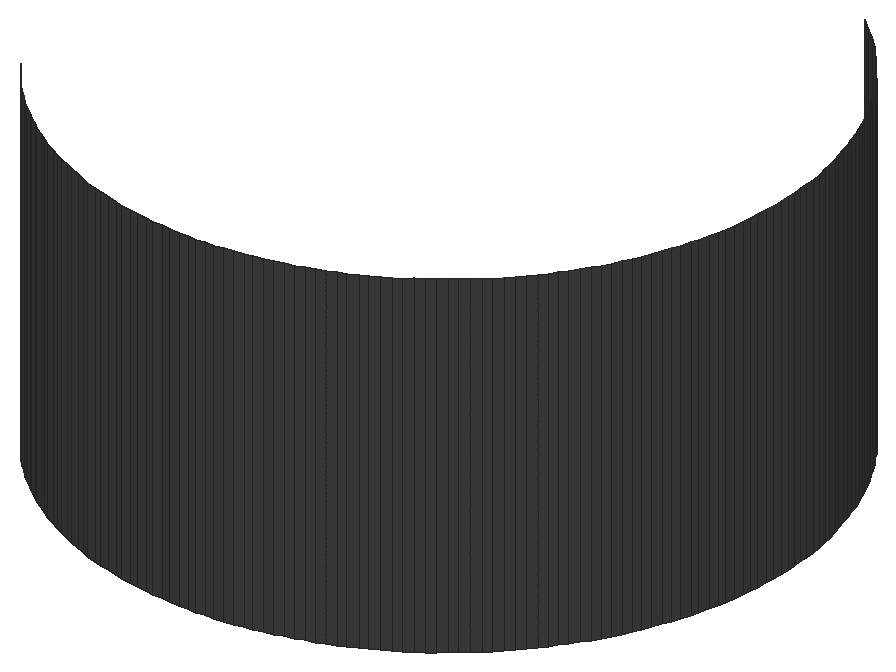
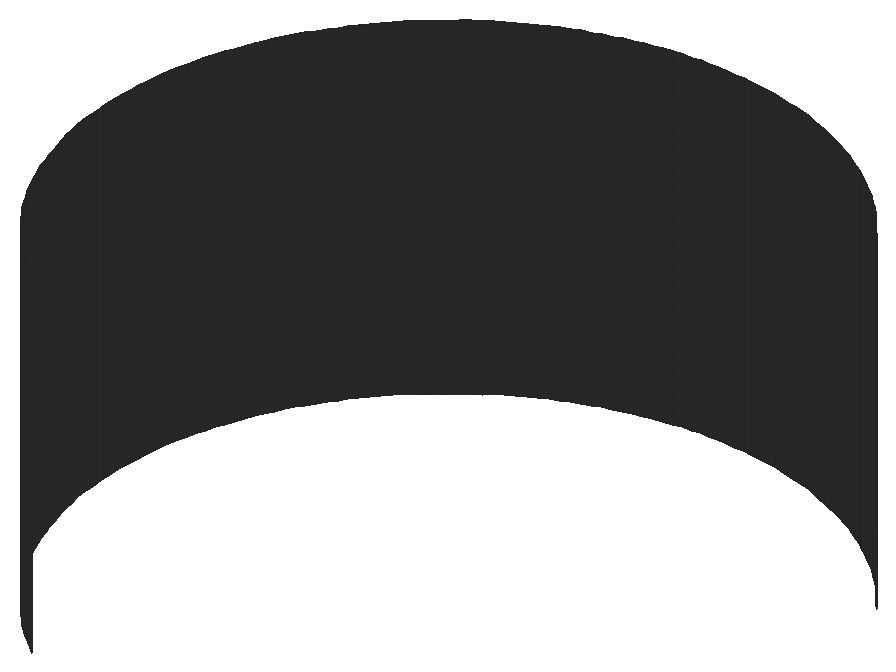
# SketchUp Ruby script. Lengths in inches.
U = 1.inch
M = Sketchup.active_model
def pt(a) = Geom::Point3d.new(a.map { |v| v * U })
def face(e, loops, mat)
  f = e.add_face(loops[0].map { |a| pt(a) })
  loops[1..].each { |l| e.add_face(l.map { |a| pt(a) }).erase! }
  f.material = f.back_material = mat if mat
  f
end
# faces: each face lists its corners as indices into pts; further lists are holes
def faces(e, pts, list, mat = nil) = list.each { |f| face(e, (f[0].is_a?(Array) ? f : [f]).map { |l| l.map { |i| pts[i] } }, mat) }
# xy, xz, yz: faces in a plane at the given z, y or x. An outline is a flat list of corners, or four numbers for a rectangle; further outlines are holes
def ring(l) = l.size == 4 ? [[l[0], l[1]], [l[2], l[1]], [l[2], l[3]], [l[0], l[3]]] : l.each_slice(2).to_a
def flat(e, list, mat, &to3) = list.each { |f| face(e, (f[0].is_a?(Array) ? f : [f]).map { |l| ring(l).map { |u, v| to3.(u, v) } }, mat) }
def xy(e, z, list, mat = nil) = flat(e, list, mat) { |x, y| [x, y, z] }
def xz(e, y, list, mat = nil) = flat(e, list, mat) { |x, z| [x, y, z] }
def yz(e, x, list, mat = nil) = flat(e, list, mat) { |y, z| [x, y, z] }
def lines(e, pts, list) = list.each { |a, b| e.add_line(pt(pts[a]), pt(pts[b])) }
# prism: a flat outline (further loops are holes) pulled along v
def prism(e, loops, v, mat = nil)
  f = face(e, loops, mat); d = Geom::Vector3d.new(v.map { |x| x * U })
  f.pushpull(f.normal.samedirection?(d) ? d.length : -d.length)
end
def box(e, o, s, mat = nil) = prism(e, [[o, [o[0] + s[0], o[1], o[2]], [o[0] + s[0], o[1] + s[1], o[2]], [o[0], o[1] + s[1], o[2]]]], [0, 0, s[2]], mat)
def at(x, y, z, deg = 0) = Geom::Transformation.translation(pt([x, y, z])) * Geom::Transformation.rotation(ORIGIN, Z_AXIS, deg.degrees)
def axes(o, x, y, z) = Geom::Transformation.new([*x, 0, *y, 0, *z, 0, *pt(o).to_a, 1])
def part(name) = M.definitions.add(name)
# library, detail: a bought-in or finely detailed component or shape, given as its bounding box
def library(name, o, s) = part(name).tap { |d| box(d.entities, o, s) }
def detail(e, o, s) = box(e.add_group.entities, o, s)
def put(e, d, t, mat = nil) = e.add_instance(d, t).tap { |i| i.material = mat if mat }
def group(e, t, mat = nil) = e.add_group.tap { |g| g.transformation = t; g.material = mat if mat }.entities
root = M.entities
M.materials.add("1448 AP 8253 RAVEN SONG").color = [64, 64, 63]
xz(root,204,[[39.35,120,39.43,123],[39.43,120,39.51,123],[39.51,120,39.59,123]],"1448 AP 8253 RAVEN SONG")
xz(root,204.01,[[39.19,120,39.27,123],[39.66,120,39.74,123]],"1448 AP 8253 RAVEN SONG")
yz(root,42.45,[[206.9,120,206.98,123],[206.98,120,207.06,123],[207.06,120,207.14,123]],"1448 AP 8253 RAVEN SONG")
p = [[38.96,204.04,120],[38.88,204.05,120],[38.88,204.05,123],[38.96,204.04,123],[39.12,204.02,120],[39.04,204.03,120],
  [39.04,204.03,123],[39.12,204.02,123],[39.19,204.01,120],[39.19,204.01,123],[39.35,204,120],[39.27,204.01,120],
  [39.27,204.01,123],[39.35,204,123],[39.66,204.01,120],[39.59,204,120],[39.59,204,123],[39.66,204.01,123],
  [39.82,204.02,120],[39.74,204.01,120],[39.74,204.01,123],[39.82,204.02,123],[39.9,204.03,120],[39.9,204.03,123],
  [39.98,204.05,120],[39.98,204.05,123],[40.05,204.0625,120],[40.05,204.0625,123],[38.58,204.13,120],[38.5,204.15,120],
  [38.5,204.15,123],[38.58,204.13,123],[38.65,204.11,120],[38.65,204.11,123],[38.81,204.07,120],[38.73,204.09,120],
  [38.73,204.09,123],[38.81,204.07,123],[40.21,204.1,120],[40.13,204.08,120],[40.13,204.08,123],[40.21,204.1,123],
  [40.28,204.12,120],[40.28,204.12,123],[40.36,204.14,120],[40.36,204.14,123],[40.43,204.17,120],[40.43,204.17,123],
  [38.28,204.24,120],[38.21,204.27,120],[38.21,204.27,123],[38.28,204.24,123],[38.36,204.21,120],[38.36,204.21,123],
  [38.43,204.18,120],[38.43,204.18,123],[40.51,204.19,120],[40.51,204.19,123],[40.58,204.22,120],[40.58,204.22,123],
  [40.65,204.25,120],[40.65,204.25,123],[38.07,204.34,120],[38,204.375,120],[38,204.375,123],[38.07,204.34,123],
  [38.14,204.3,120],[38.14,204.3,123],[40.79,204.32,120],[40.72,204.28,120],[40.72,204.28,123],[40.79,204.32,123],
  [40.86,204.35,120],[40.86,204.35,123],[37.93,204.41,120],[37.93,204.41,123],[37.87,204.45,120],[37.87,204.45,123],
  [41,204.43,120],[40.93,204.39,120],[40.93,204.39,123],[41,204.43,123],[41.07,204.47,120],[41.07,204.47,123],
  [37.8,204.5,120],[37.73,204.54,120],[37.73,204.54,123],[37.8,204.5,123],[37.67,204.59,120],[37.67,204.59,123],
  [41.2,204.5625,120],[41.13,204.52,120],[41.13,204.52,123],[41.2,204.5625,123],[37.61,204.63,120],[37.55,204.68,120],
  [37.55,204.68,123],[37.61,204.63,123],[41.26,204.61,120],[41.26,204.61,123],[41.32,204.66,120],[41.32,204.66,123],
  [37.49,204.73,120],[37.43,204.78,120],[37.43,204.78,123],[37.49,204.73,123],[41.38,204.71,120],[41.38,204.71,123],
  [41.44,204.76,120],[41.44,204.76,123],[37.37,204.84,120],[37.3125,204.89,120],[37.3125,204.89,123],[37.37,204.84,123],
  [41.5,204.81,120],[41.5,204.81,123],[41.56,204.86,120],[41.56,204.86,123],[37.26,204.95,120],[37.21,205.01,120],
  [37.21,205.01,123],[37.26,204.95,123],[41.67,204.98,120],[41.61,204.92,120],[41.61,204.92,123],[41.67,204.98,123],
  [37.16,205.07,120],[37.16,205.07,123],[41.77,205.1,120],[41.72,205.04,120],[41.72,205.04,123],[41.77,205.1,123],
  [37.11,205.13,120],[37.11,205.13,123],[37.06,205.19,120],[37.06,205.19,123],[41.82,205.16,120],[41.82,205.16,123],
  [41.86,205.22,120],[41.86,205.22,123],[41.91,205.28,120],[41.91,205.28,123],[41.95,205.35,120],[41.95,205.35,123],
  [42,205.42,120],[42,205.42,123],[42.04,205.48,120],[42.04,205.48,123],[42.08,205.55,120],[42.08,205.55,123],
  [42.15,205.69,120],[42.11,205.62,120],[42.11,205.62,123],[42.15,205.69,123],[42.18,205.76,120],[42.18,205.76,123],
  [42.24,205.91,120],[42.21,205.83,120],[42.21,205.83,123],[42.24,205.91,123],[42.27,205.98,120],[42.27,205.98,123],
  [42.3,206.05,120],[42.3,206.05,123],[42.34,206.2,120],[42.32,206.13,120],[42.32,206.13,123],[42.34,206.2,123],
  [42.36,206.28,120],[42.36,206.28,123],[42.38,206.36,120],[42.38,206.36,123],[42.41,206.51,120],[42.4,206.43,120],
  [42.4,206.43,123],[42.41,206.51,123],[42.42,206.59,120],[42.42,206.59,123],[42.43,206.67,120],[42.43,206.67,123],
  [42.44,206.82,120],[42.4375,206.74,120],[42.4375,206.74,123],[42.44,206.82,123],[42.45,206.9,120],[42.45,206.9,123],
  [42.44,207.21,120],[42.45,207.14,120],[42.45,207.14,123],[42.44,207.21,123],[42.4375,207.29,120],[42.4375,207.29,123],
  [42.43,207.37,120],[42.43,207.37,123],[42.4,207.53,120],[42.42,207.45,120],[42.42,207.45,123],[42.4,207.53,123],
  [42.39,207.6,120],[42.39,207.6,123],[42.37,207.68,120],[42.37,207.68,123],[42.35,207.76,120],[42.35,207.76,123],
  [42.31,207.91,120],[42.33,207.83,120],[42.33,207.83,123],[42.31,207.91,123],[42.28,207.98,120],[42.28,207.98,123],
  [42.26,208.06,120],[42.26,208.06,123],[42.2,208.2,120],[42.23,208.13,120],[42.23,208.13,123],[42.2,208.2,123],
  [42.17,208.27,120],[42.17,208.27,123],[42.1,208.41,120],[42.13,208.34,120],[42.13,208.34,123],[42.1,208.41,123],
  [42.06,208.48,120],[42.06,208.48,123],[41.98,208.62,120],[42.02,208.55,120],[42.02,208.55,123],[41.98,208.62,123],
  [41.93,208.68,120],[41.93,208.68,123],[41.84,208.81,120],[41.89,208.75,120],[41.89,208.75,123],[41.84,208.81,123],
  [41.79,208.87,120],[41.79,208.87,123],[41.69,208.99,120],[41.74,208.93,120],[41.74,208.93,123],[41.69,208.99,123],
  [41.64,209.05,120],[41.64,209.05,123],[41.53,209.16,120],[41.59,209.11,120],[41.59,209.11,123],[41.53,209.16,123],
  [41.41,209.27,120],[41.47,209.22,120],[41.47,209.22,123],[41.41,209.27,123],[41.29,209.37,120],[41.35,209.32,120],
  [41.35,209.32,123],[41.29,209.37,123]]
faces(root,p,[[0,1,2,3],[4,5,6,7],[5,0,3,6],[8,4,7,9],[10,11,12,13],[14,15,16,17],[18,19,20,21],[22,18,21,23],
  [24,22,23,25],[26,24,25,27],[28,29,30,31],[32,28,31,33],[34,35,36,37],[35,32,33,36],[1,34,37,2],[38,39,40,41],
  [39,26,27,40],[42,38,41,43],[44,42,43,45],[46,44,45,47],[48,49,50,51],[52,48,51,53],[29,54,55,30],[54,52,53,55],
  [56,46,47,57],[58,56,57,59],[60,58,59,61],[62,63,64,65],[49,66,67,50],[66,62,65,67],[68,69,70,71],[69,60,61,70],
  [72,68,71,73],[63,74,75,64],[74,76,77,75],[78,79,80,81],[79,72,73,80],[82,78,81,83],[84,85,86,87],[85,88,89,86],
  [76,84,87,77],[90,91,92,93],[91,82,83,92],[94,95,96,97],[88,94,97,89],[98,90,93,99],[100,98,99,101],[102,103,104,105],
  [95,102,105,96],[106,100,101,107],[108,106,107,109],[110,111,112,113],[103,110,113,104],[114,108,109,115],[116,114,115,117],[118,119,120,121],
  [111,118,121,112],[122,123,124,125],[123,116,117,124],[119,126,127,120],[128,129,130,131],[129,122,125,130],[126,132,133,127],[132,134,135,133],
  [136,128,131,137],[138,136,137,139],[140,138,139,141],[142,140,141,143],[144,142,143,145],[146,144,145,147],[148,146,147,149],[150,151,152,153],
  [151,148,149,152],[154,150,153,155],[156,157,158,159],[157,154,155,158],[160,156,159,161],[162,160,161,163],[164,165,166,167],[165,162,163,166],
  [168,164,167,169],[170,168,169,171],[172,173,174,175],[173,170,171,174],[176,172,175,177],[178,176,177,179],[180,181,182,183],[181,178,179,182],
  [184,180,183,185],[186,187,188,189],[190,186,189,191],[192,190,191,193],[194,195,196,197],[195,192,193,196],[198,194,197,199],[200,198,199,201],
  [202,200,201,203],[204,205,206,207],[205,202,203,206],[208,204,207,209],[210,208,209,211],[212,213,214,215],[213,210,211,214],[216,212,215,217],
  [218,219,220,221],[219,216,217,220],[222,218,221,223],[224,225,226,227],[225,222,223,226],[228,224,227,229],[230,231,232,233],[231,228,229,232],
  [234,230,233,235],[236,237,238,239],[237,234,235,238],[240,236,239,241],[242,243,244,245],[243,240,241,244],[246,247,248,249],[247,242,245,248],
  [250,251,252,253],[251,246,249,252]],"1448 AP 8253 RAVEN SONG")
